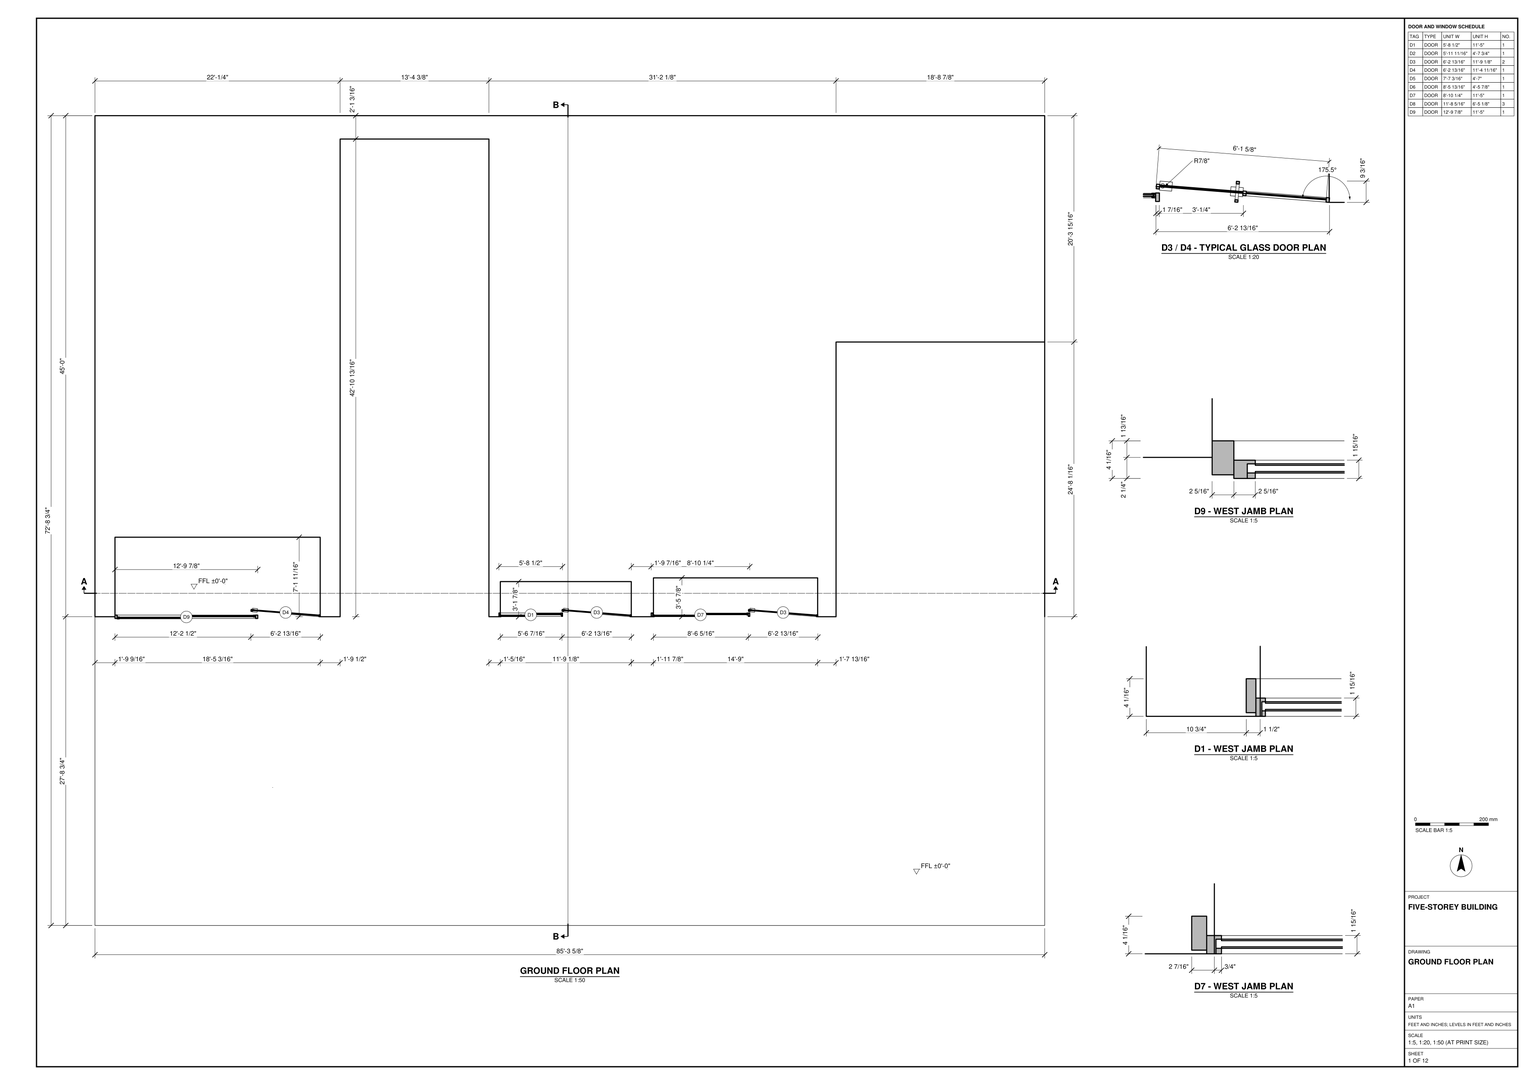
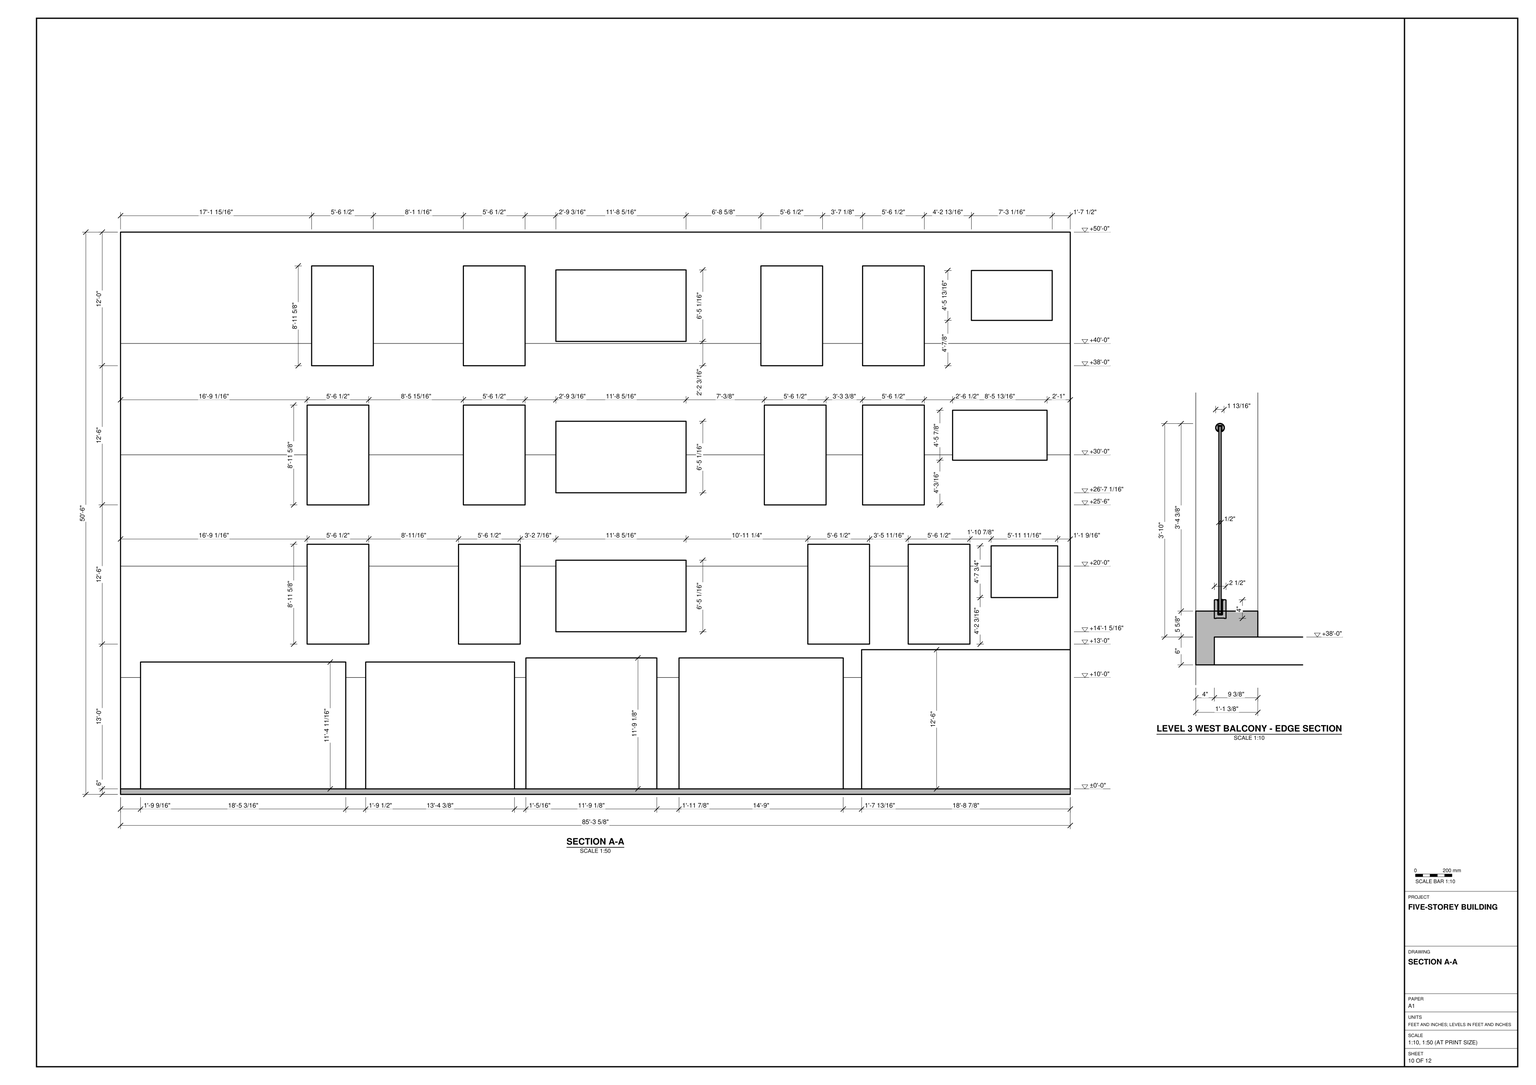
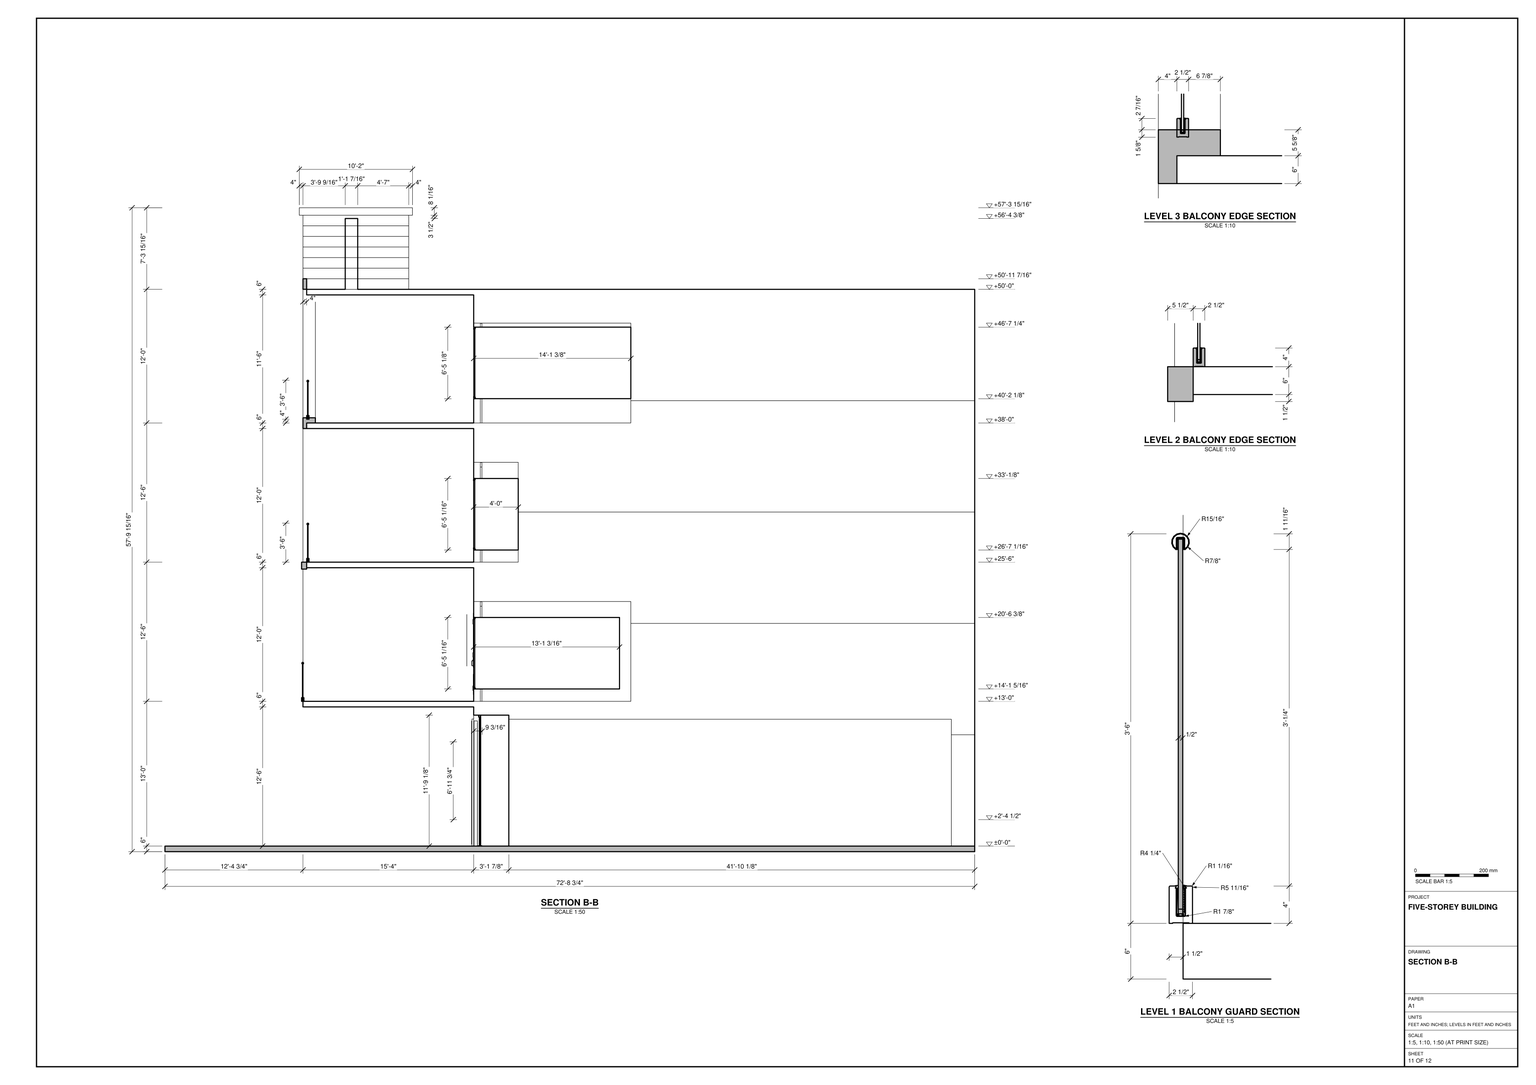
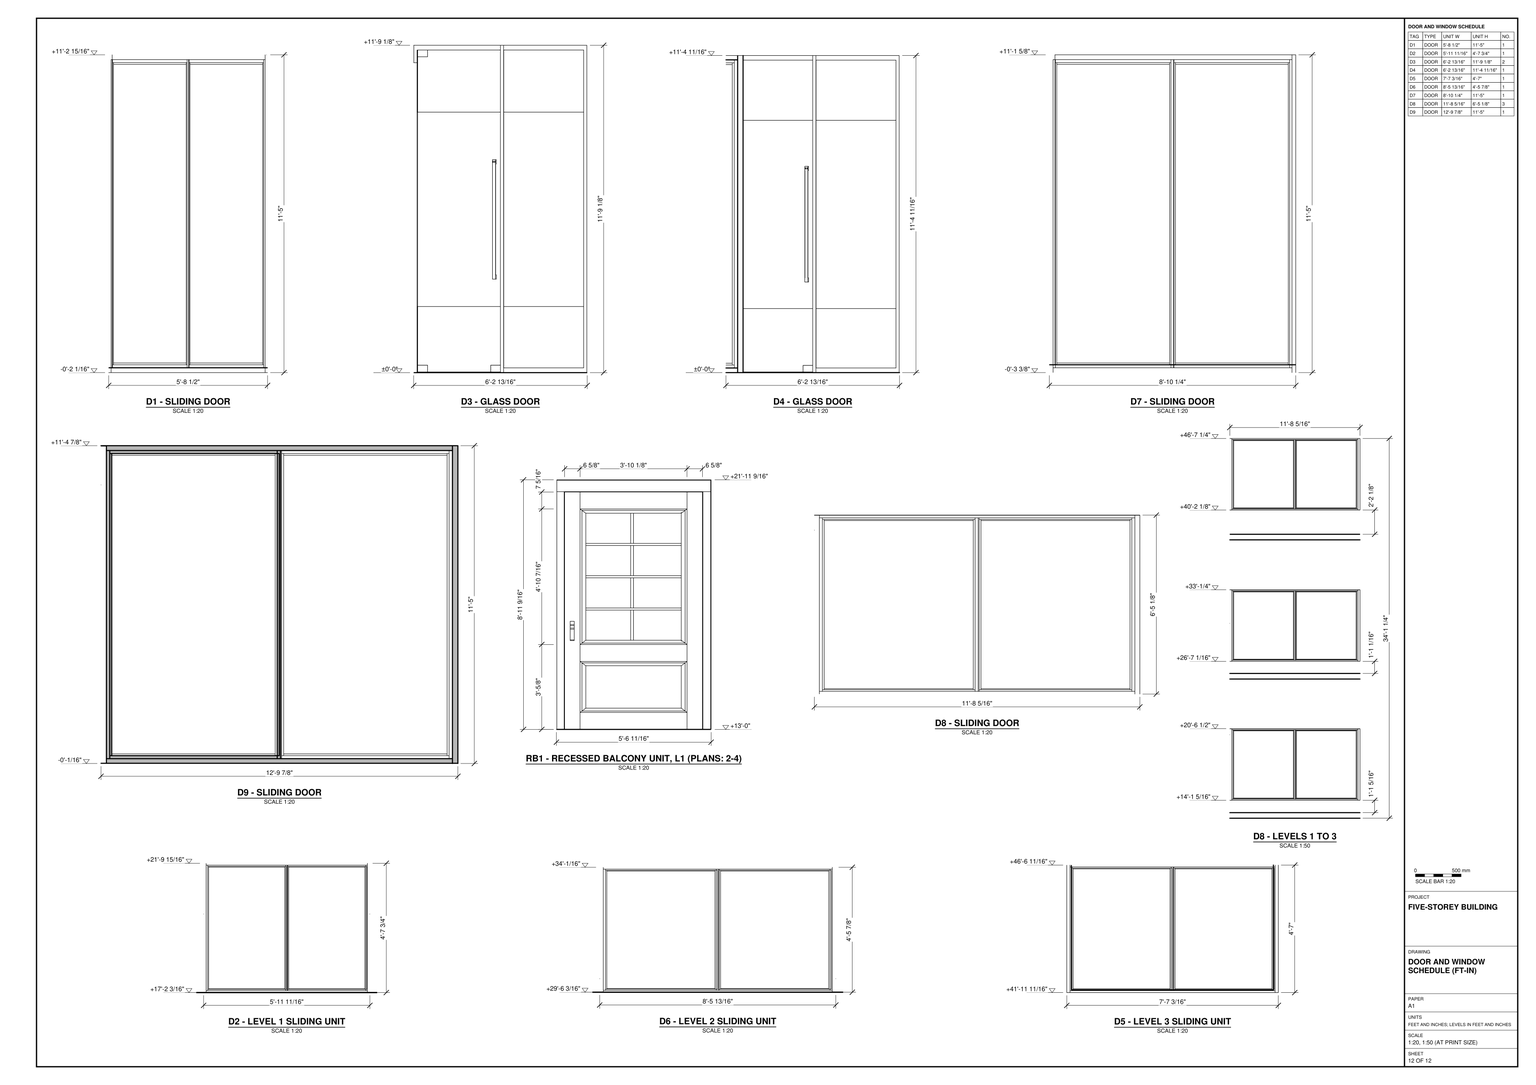
Build the five-storey building in SketchUp from task_files/diagram_01.pdf. Work in feet and inches. The overall model extents are 85'-7 5/8" along X, 72'-8 3/4" along Y and 57'-9 15/16" along Z. Set the ground floor at ±0'-0" and the successive levels at +13'-0", +25'-6", +38'-0" and +50'-0".

Start with the rectangular ground slab. Trace the stepped ground-floor footprint, preserving the deep recess between the entrance bays and the setback at the east end. Model the walls at their drawn thicknesses and fit the glazed door assemblies to the openings using the plan and jamb details. Use section A-A to locate the tall openings and the wider horizontal openings on each upper floor rather than repeating an identical layout. Use section B-B and the enlarged details to shape the projecting balcony slabs, their edges and their glass guards. Include the roof slab and the capped structure rising above it. Follow the plans for any stairs, built-in joinery and main furniture shown.

Keep shell elements and each furniture or joinery piece in separate groups or components, and use components for repeated parts. Decor and loose items may be any suitable library components. Save one SketchUp model as output_files/five_storey_building_with_glazed_entries_and_balconies.skp.

# SketchUp Ruby script. Lengths in inches.
U = 1.inch
M = Sketchup.active_model
def pt(a) = Geom::Point3d.new(a.map { |v| v * U })
def face(e, loops, mat)
  f = e.add_face(loops[0].map { |a| pt(a) })
  loops[1..].each { |l| e.add_face(l.map { |a| pt(a) }).erase! }
  f.material = f.back_material = mat if mat
  f
end
# faces: each face lists its corners as indices into pts; further lists are holes
def faces(e, pts, list, mat = nil) = list.each { |f| face(e, (f[0].is_a?(Array) ? f : [f]).map { |l| l.map { |i| pts[i] } }, mat) }
# xy, xz, yz: faces in a plane at the given z, y or x. An outline is a flat list of corners, or four numbers for a rectangle; further outlines are holes
def ring(l) = l.size == 4 ? [[l[0], l[1]], [l[2], l[1]], [l[2], l[3]], [l[0], l[3]]] : l.each_slice(2).to_a
def flat(e, list, mat, &to3) = list.each { |f| face(e, (f[0].is_a?(Array) ? f : [f]).map { |l| ring(l).map { |u, v| to3.(u, v) } }, mat) }
def xy(e, z, list, mat = nil) = flat(e, list, mat) { |x, y| [x, y, z] }
def xz(e, y, list, mat = nil) = flat(e, list, mat) { |x, z| [x, y, z] }
def yz(e, x, list, mat = nil) = flat(e, list, mat) { |y, z| [x, y, z] }
def lines(e, pts, list) = list.each { |a, b| e.add_line(pt(pts[a]), pt(pts[b])) }
# prism: a flat outline (further loops are holes) pulled along v
def prism(e, loops, v, mat = nil)
  f = face(e, loops, mat); d = Geom::Vector3d.new(v.map { |x| x * U })
  f.pushpull(f.normal.samedirection?(d) ? d.length : -d.length)
end
def box(e, o, s, mat = nil) = prism(e, [[o, [o[0] + s[0], o[1], o[2]], [o[0] + s[0], o[1] + s[1], o[2]], [o[0], o[1] + s[1], o[2]]]], [0, 0, s[2]], mat)
def at(x, y, z, deg = 0) = Geom::Transformation.translation(pt([x, y, z])) * Geom::Transformation.rotation(ORIGIN, Z_AXIS, deg.degrees)
def axes(o, x, y, z) = Geom::Transformation.new([*x, 0, *y, 0, *z, 0, *pt(o).to_a, 1])
def part(name) = M.definitions.add(name)
# library, detail: a bought-in or finely detailed component or shape, given as its bounding box
def library(name, o, s) = part(name).tap { |d| box(d.entities, o, s) }
def detail(e, o, s) = box(e.add_group.entities, o, s)
def put(e, d, t, mat = nil) = e.add_instance(d, t).tap { |i| i.material = mat if mat }
def group(e, t, mat = nil) = e.add_group.tap { |g| g.transformation = t; g.material = mat if mat }.entities
root = M.entities
M.materials.add("Color_B03").color = [113, 96, 78]
M.materials.add("Glass_Tinted_Gray").color = [0, 0, 0]
M.materials["Glass_Tinted_Gray"].alpha = 0.125
M.materials.add("[0135_DarkGray]").color = [81, 81, 81]
M.materials.add("[Color_007]").color = [58, 58, 58]
M.materials.add("[Color_C10]").color = [204, 183, 163]
M.materials.add("[Color_E22]").color = [51, 51, 10]
M.materials.add("[Mirror 02]").color = [229, 229, 229]
M.materials.add("[Terrazzo Light Blue]").color = [196, 214, 227]
M.materials.add("[Wood Floor Parquet]").color = [145, 89, 39]
M.materials.add("[Wood Veneer 01]").color = [120, 70, 37]
c1 = part("Door frame head")
box(c1.entities,[24,0,0],[40,1.75,4],"[Color_C10]")
c2 = part("Door jamb")
box(c2.entities,[0,0,0],[2,1.75,84],"[Color_C10]")
c3 = part("Door panel moulding")
xy(c3.entities,0,[[0,0,47.875,0.25],[0,2,47.875,2.25]],"[Color_C10]")
xy(c3.entities,1.5,[[1.5,0.25,46.375,2]],"[Color_C10]")
xz(c3.entities,0,[[0,0,47.875,0,47.375,0.5,0.5,0.5]],"[Color_C10]")
xz(c3.entities,2.25,[[0,0,0.5,0.5,47.375,0.5,47.875,0]],"[Color_C10]")
p = [[46.375,0.25,1.5],[1.5,0.25,1.5],[0.5,0,0.5],[47.375,0,0.5],[1.5,2,1.5],[46.375,2,1.5],
  [47.375,2.25,0.5],[0.5,2.25,0.5]]
faces(c3.entities,p,[[0,1,2,3],[4,5,6,7]],"[Color_C10]")
c4 = part("Hinge plate")
box(c4.entities,[0,0,0],[0.125,2.5,4],"[Color_E22]")
c5 = part("Door panel moulding \#1")
xy(c5.entities,0,[[0,0,27.75,0.25],[0,2,27.75,2.25]],"[Color_C10]")
xy(c5.entities,1.5,[[1.5,0.25,26.25,2]],"[Color_C10]")
xz(c5.entities,0,[[0,0,27.75,0,27.25,0.5,0.5,0.5]],"[Color_C10]")
xz(c5.entities,2.25,[[0,0,0.5,0.5,27.25,0.5,27.75,0]],"[Color_C10]")
p = [[26.25,0.25,1.5],[1.5,0.25,1.5],[0.5,0,0.5],[27.25,0,0.5],[27.25,2.25,0.5],[0.5,2.25,0.5],
  [1.5,2,1.5],[26.25,2,1.5]]
faces(c5.entities,p,[[0,1,2,3],[4,5,6,7]],"[Color_C10]")
c6 = part("Door pull handle")
xy(c6.entities,0,[[0,0.24,1.05,1.04]],"[Color_E22]")
xy(c6.entities,0.3,[[0,0.64,1.05,1.04]],"[Color_E22]")
xy(c6.entities,6.83,[[0,1.4375,1.05,1.875]],"[Color_E22]")
xz(c6.entities,0,[[0,0.24,1.05,4.01]],"[Color_E22]")
xz(c6.entities,0.39,[[0,0.55,1.05,3.59]],"[Color_E22]")
xz(c6.entities,1.17,[[0,0.07,1.05,0.22]],"[Color_E22]")
xz(c6.entities,1.4375,[[0,5.64,1.05,6.83]],"[Color_E22]")
yz(c6.entities,0,[[0.24,0,0.12,0.03,0.03,0.12,0,0.24,0,4.01,0.02,4.17,0.09,4.31,0.2,4.43,1.28,5.31,1.36,5.4,1.42,5.52,1.4375,5.64,1.4375,6.83,1.875,6.83,1.875,5.29,1.86,5.18,1.81,5.08,1.73,5,0.7,4.22,0.53,4.05,0.43,3.83,0.39,3.59,0.39,0.55,0.42,0.42,0.52,0.33,0.64,0.3,1.04,0.3,1.17,0.22,1.17,0.07,1.04,0]],"[Color_E22]")
yz(c6.entities,1.05,[[0.24,0,1.04,0,1.17,0.07,1.17,0.22,1.04,0.3,0.64,0.3,0.52,0.33,0.42,0.42,0.39,0.55,0.39,3.59,0.43,3.83,0.53,4.05,0.7,4.22,1.73,5,1.81,5.08,1.86,5.18,1.875,5.29,1.875,6.83,1.4375,6.83,1.4375,5.64,1.42,5.52,1.36,5.4,1.28,5.31,0.2,4.43,0.09,4.31,0.02,4.17,0,4.01,0,0.24,0.03,0.12,0.12,0.03]],"[Color_E22]")
p = [[0,0.03,0.12],[0,0.12,0.03],[1.05,0.12,0.03],[1.05,0.03,0.12],[0,0.24,0],[1.05,0.24,0],
  [1.05,1.17,0.07],[1.05,1.04,0],[0,1.04,0],[0,1.17,0.07],[0,0,0.24],[1.05,0,0.24],
  [1.05,1.04,0.3],[1.05,1.17,0.22],[0,1.17,0.22],[0,1.04,0.3],[0,0.52,0.33],[0,0.42,0.42],
  [1.05,0.42,0.42],[1.05,0.52,0.33],[0,0.64,0.3],[1.05,0.64,0.3],[0,0.39,0.55],[1.05,0.39,0.55],
  [0,0.39,3.59],[0,0.43,3.83],[1.05,0.43,3.83],[1.05,0.39,3.59],[0,0.53,4.05],[1.05,0.53,4.05],
  [0,0.02,4.17],[0,0,4.01],[1.05,0,4.01],[1.05,0.02,4.17],[0,0.7,4.22],[1.05,0.7,4.22],
  [0,0.09,4.31],[1.05,0.09,4.31],[0,1.73,5],[1.05,1.73,5],[0,0.2,4.43],[1.05,0.2,4.43],
  [1.05,1.28,5.31],[0,1.28,5.31],[1.05,1.81,5.08],[0,1.81,5.08],[1.05,1.86,5.18],[0,1.86,5.18],
  [1.05,1.875,5.29],[0,1.875,5.29],[0,1.36,5.4],[1.05,1.36,5.4],[0,1.42,5.52],[1.05,1.42,5.52],
  [0,1.4375,5.64],[1.05,1.4375,5.64]]
faces(c6.entities,p,[[0,1,2,3],[1,4,5,2],[6,7,8,9],[10,0,3,11],[12,13,14,15],[16,17,18,19],[20,16,19,21],[17,22,23,18],
  [24,25,26,27],[25,28,29,26],[30,31,32,33],[28,34,35,29],[36,30,33,37],[34,38,39,35],[40,36,37,41],[40,41,42,43],
  [44,39,38,45],[46,44,45,47],[48,46,47,49],[50,43,42,51],[52,50,51,53],[54,52,53,55]],"[Color_E22]")
c7 = part("Component\#153")
xz(c7.entities,0,[[0,6,27.75,53.875]],"[Color_007]")
c8 = part("Door panel moulding \#2")
xy(c8.entities,0,[[35.875,0,53.875,0.25],[35.875,2,53.875,2.25]],"[Color_C10]")
xy(c8.entities,1.5,[[37.375,0.25,52.375,2]],"[Color_C10]")
xz(c8.entities,0,[[35.875,0,53.875,0,53.375,0.5,36.375,0.5]],"[Color_C10]")
xz(c8.entities,2.25,[[35.875,0,36.375,0.5,53.375,0.5,53.875,0]],"[Color_C10]")
p = [[52.375,0.25,1.5],[37.375,0.25,1.5],[36.375,0,0.5],[53.375,0,0.5],[37.375,2,1.5],[52.375,2,1.5],
  [53.375,2.25,0.5],[36.375,2.25,0.5]]
faces(c8.entities,p,[[0,1,2,3],[4,5,6,7]],"[Color_C10]")
c9 = part("Door stile")
box(c9.entities,[0,0,0],[4,1.75,83.875],"[Color_C10]")
c10 = part("Lower door panel")
box(c10.entities,[0,0,0],[27.75,1.75,30],"[Color_C10]")
c11 = part("Door panel moulding \#3")
xy(c11.entities,0,[[0,0,27.75,0.25],[0,2,27.75,2.25]],"[Color_C10]")
xy(c11.entities,1.5,[[1.5,0.25,26.25,2]],"[Color_C10]")
xz(c11.entities,0,[[0,0,27.75,0,27.25,0.5,0.5,0.5]],"[Color_C10]")
xz(c11.entities,2.25,[[0,0,0.5,0.5,27.25,0.5,27.75,0]],"[Color_C10]")
p = [[26.25,0.25,1.5],[1.5,0.25,1.5],[0.5,0,0.5],[27.25,0,0.5],[27.25,2.25,0.5],[0.5,2.25,0.5],
  [1.5,2,1.5],[26.25,2,1.5]]
faces(c11.entities,p,[[0,1,2,3],[4,5,6,7]],"[Color_C10]")
c12 = part("Door rail")
box(c12.entities,[0,0,0],[27.75,1.75,6],"[Color_C10]")
c13 = part("Horizontal glazing bar")
xy(c13.entities,0,[[0,0,24.75,1.75]],"[Color_C10]")
xy(c13.entities,0.75,[[0,0,24.75,1.75]],"[Color_C10]")
xz(c13.entities,0,[[0,0,24.75,0.75]],"[Color_C10]")
xz(c13.entities,1.75,[[0,0,24.75,0.75]],"[Color_C10]")
c14 = part("Vertical glazing bar")
xz(c14.entities,0,[[0,6,0.75,16.66],[0,17.41,0.75,28.0625],[0,28.8125,0.75,39.47],[0,40.22,0.75,50.875]],"[Color_C10]")
xz(c14.entities,1.75,[[0,6,0.75,16.66],[0,17.41,0.75,28.0625],[0,28.8125,0.75,39.47],[0,40.22,0.75,50.875]],"[Color_C10]")
yz(c14.entities,0,[[0,6,1.75,16.66],[0,17.41,1.75,28.0625],[0,28.8125,1.75,39.47],[0,40.22,1.75,50.875]],"[Color_C10]")
yz(c14.entities,0.75,[[0,6,1.75,16.66],[0,17.41,1.75,28.0625],[0,28.8125,1.75,39.47],[0,40.22,1.75,50.875]],"[Color_C10]")
c15 = part("Glazed door leaf")
p = [[5.625,-5.28,31.125],[5.625,-5.28,42.53],[5.625,-5.28,53.9375],[5.625,-5.28,65.34],[5.625,-5.28,76.75]]
lines(c15.entities,p,[[0,1],[1,2],[2,3],[3,4]])
put(c15.entities,c3,axes([4.125,1.625,77.875],[0,0,-1],[0,1,0],[1,0,0]))
put(c15.entities,c4,at(0,1.125,68.3))
put(c15.entities,c5,at(4.125,1.625,6))
put(c15.entities,c6,at(33.38,0,31.375))
put(c15.entities,c7,at(4.125,2.75,24))
put(c15.entities,c8,axes([31.875,1.625,59.875],[0,0,-1],[0,1,0],[-1,0,0]))
put(c15.entities,c9,at(31.875,1.875,0))
put(c15.entities,c8,axes([4.125,1.625,59.875],[0,0,-1],[0,1,0],[1,0,0]))
put(c15.entities,c10,at(4.125,1.875,0))
put(c15.entities,c11,axes([4.125,1.625,77.875],[1,0,0],[0,1,0],[0,0,-1]))
put(c15.entities,c3,axes([31.875,1.625,77.875],[0,0,-1],[0,1,0],[-1,0,0]))
put(c15.entities,c11,at(4.125,1.625,30))
put(c15.entities,c12,at(4.125,1.875,77.875))
put(c15.entities,c9,at(0.125,1.875,0))
put(c15.entities,c13,at(5.625,1.875,42.16))
put(c15.entities,c14,at(18,1.875,25.5))
put(c15.entities,c4,at(0,1.125,9.62))
put(c15.entities,c5,axes([4.125,1.625,24],[1,0,0],[0,1,0],[0,0,-1]))
put(c15.entities,c4,at(0,1.125,38.96))
put(c15.entities,c13,at(5.625,1.875,53.5625))
put(c15.entities,c13,at(5.625,1.875,64.97))
c16 = part("Glazed door assembly")
put(c16.entities,c1,at(-30,0,84))
put(c16.entities,c2,at(32,0,0))
put(c16.entities,c2,at(-6,0,0))
put(c16.entities,c15,axes([32,-1.875,0],[-1,0,0],[0,1,0],[0,0,1]))
c17 = part("PENTEK_RP Fineline 50S_Sliding_DoorCase_E1")
box(c17.entities,[0,0,0],[1.51,3.66,99.27],"[0135_DarkGray]")
c18 = part("PENTEK_RP Fineline 50S_SlidingDooe_Case_E2")
box(c18.entities,[0,0,0],[96.25,3.66,1.51],"[0135_DarkGray]")
c19 = part("pentek_RP Fineline 50S_SlidingDoor_Case")
put(c19.entities,c17,at(97.76,0,0))
put(c19.entities,c18,at(1.51,0,0))
put(c19.entities,c17,at(0,0,0))
put(c19.entities,c18,at(1.51,0,97.76))
c20 = part("PENTEK_RP Fineline 50S_SlidingDoor_GlazingBead_2")
box(c20.entities,[0,0,0],[0.56,0.59,94.39],"[0135_DarkGray]")
c21 = part("PENTEK_RP Fineline 50S_SlidingDoor_Glass")
box(c21.entities,[0,0,0],[46.58,0.16,94.39],"Glass_Tinted_Gray")
c22 = part("PENTEK_RP Fineline 50S_SlidingDoor_GlazingBead")
box(c22.entities,[0,0,0],[45.47,0.59,0.56],"[0135_DarkGray]")
c23 = part("PENTEK_RP Fineline 50S_SlidingDoor_Leaf_E1")
xy(c23.entities,0,[[0,0,0.93,1.97],[0.93,1.57,1.49,1.97]],"[0135_DarkGray]")
xy(c23.entities,96.25,[[0,0,0.93,0,0.93,1.57,1.49,1.57,1.49,1.97,0,1.97]],"[0135_DarkGray]")
xz(c23.entities,0,[[0,0,0.93,96.25]],"[0135_DarkGray]")
xz(c23.entities,1.57,[[0.93,0,1.49,95.32],[0.93,95.32,1.49,96.25]],"[0135_DarkGray]")
xz(c23.entities,1.97,[[0,0,1.49,96.25]],"[0135_DarkGray]")
yz(c23.entities,0,[[0,0,1.97,96.25]],"[0135_DarkGray]")
yz(c23.entities,0.93,[[0,0,1.57,0.93],[0,0.93,1.57,95.32],[0,95.32,1.57,96.25]],"[0135_DarkGray]")
yz(c23.entities,1.49,[[1.57,0,1.97,95.32],[1.57,95.32,1.97,96.25]],"[0135_DarkGray]")
c24 = part("PENTEK_RP Fineline 50S_SlidingDoor_Leaf_E2")
xy(c24.entities,0,[[0,0,0,1.57,0.56,1.57,0.56,1.97,46.02,1.97,46.02,1.57,46.58,1.57,46.58,0]],"[0135_DarkGray]")
xy(c24.entities,0.93,[[0,0,46.58,1.57]],"[0135_DarkGray]")
xy(c24.entities,1.49,[[0.56,1.57,46.02,1.97]],"[0135_DarkGray]")
xz(c24.entities,0,[[0,0,46.58,0.93]],"[0135_DarkGray]")
xz(c24.entities,1.57,[[0,0,0.56,0.93],[46.02,0,46.58,0.93],[0.56,0.93,46.02,1.49]],"[0135_DarkGray]")
xz(c24.entities,1.97,[[0.56,0,46.02,1.49]],"[0135_DarkGray]")
yz(c24.entities,0,[[0,0,1.57,0.93]],"[0135_DarkGray]")
yz(c24.entities,0.56,[[1.57,0,1.97,0.93],[1.57,0.93,1.97,1.49]],"[0135_DarkGray]")
yz(c24.entities,46.02,[[1.57,0,1.97,0.93],[1.57,0.93,1.97,1.49]],"[0135_DarkGray]")
yz(c24.entities,46.58,[[0,0,1.57,0.93]],"[0135_DarkGray]")
c25 = part("PENTEK_RP Fineline S_SlidingDoor_Leaf1")
put(c25.entities,c20,at(0.93,0,0.93))
put(c25.entities,c20,at(46.96,0,0.93))
put(c25.entities,c21,at(1.49,1.42,0.93))
put(c25.entities,c22,at(1.49,0,0.93))
put(c25.entities,c21,at(1.49,0.59,0.93),"[Terrazzo Light Blue]")
put(c25.entities,c23,at(0,0,0))
put(c25.entities,c23,axes([48.44,0,0],[-1,0,0],[0,1,0],[0,0,1]))
put(c25.entities,c24,axes([0.93,0,96.25],[1,0,0],[0,1,0],[0,0,-1]))
put(c25.entities,c24,at(0.93,0,0))
put(c25.entities,c22,at(1.49,0,94.77))
c26 = part("PENTEK_RP Fineline 50S_SlidingDoor_Leaf2")
put(c26.entities,c21,at(1.49,1.42,0.93))
put(c26.entities,c22,at(1.49,0,94.77))
put(c26.entities,c20,at(46.96,0,0.93))
put(c26.entities,c21,at(1.49,0.59,0.93),"[Mirror 02]")
put(c26.entities,c20,at(0.93,0,0.93))
put(c26.entities,c23,at(0,0,0))
put(c26.entities,c23,axes([48.44,0,0],[-1,0,0],[0,1,0],[0,0,1]))
put(c26.entities,c22,at(1.49,0,0.93))
put(c26.entities,c24,axes([0.93,0,96.25],[1,0,0],[0,1,0],[0,0,-1]))
put(c26.entities,c24,at(0.93,0,0))
c27 = part("PENTEK - Slimmest Steel Sliding Door / Window\#1")
put(c27.entities,c19,at(0,-1.88,-0.09))
put(c27.entities,c25,at(1.51,-2.27,1.42))
put(c27.entities,c26,at(49.32,-0.3,1.42))
c28 = library("Glass Rail",[0,0,0],[2.52,48.73,42.05])
c29 = library("door glass6",[-2.49,0,0],[11.76,74.82,94.49])
xy(root,-6,[[4,0,1027.625,872.75]])
xy(root,0,[[4,0,1027.625,0,1027.625,628.8125,802.74,628.8125,802.74,332.75,782.93,332.75,782.93,374.625,605.93,374.625,605.93,332.75,582.04,332.75,582.04,370.625,440.92,370.625,440.92,332.75,428.64,332.75,428.64,847.5625,268.24,847.5625,268.24,332.75,246.74,332.75,246.74,418.4375,25.58,418.4375,25.58,332.75,4,332.75],[4,332.75,25.58,332.75,25.58,418.4375,246.74,418.4375,246.74,332.75,268.24,332.75,268.24,847.5625,428.64,847.5625,428.64,332.75,440.92,332.75,440.92,370.625,582.04,370.625,582.04,332.75,605.93,332.75,605.93,374.625,782.93,374.625,782.93,332.75,802.74,332.75,802.74,628.8125,1027.625,628.8125,1027.625,872.75,4,872.75]])
xy(root,136.6875,[[25.58,332.75,246.74,418.4375],[268.24,332.75,428.64,847.5625]])
xy(root,141.125,[[440.92,332.75,582.04,370.625],[605.93,332.75,782.93,374.625]])
xy(root,150,[[4,148.75,4,332.75,802.74,332.75,802.74,628.8125,1027.625,628.8125,1027.625,148.75]])
xy(root,156,[[535.1,147.25,544.57,148.75],[195.45,148.75,535.1,148.75,535.1,152.75,544.57,152.75,544.57,159.75,711.0625,159.75,711.0625,148.75,1017.75,148.75,1017.75,160.25,1027.625,160.25,1027.625,332.75,919.45,332.75,919.45,502.125,852.95,502.125,852.95,332.75,811.28,332.75,811.28,502.125,744.78,502.125,744.78,332.75,434.78,332.75,434.78,502.125,368.28,502.125,368.28,332.75,271.59,332.75,271.59,502.125,205.09,502.125,205.09,332.75,195.45,332.75],[535.1,148.75,544.57,152.75],[544.57,148.75,694.5,152.75],[694.5,148.75,711.0625,148.75,711.0625,159.75,544.57,159.75,544.57,152.75,694.5,152.75]])
xy(root,169.33,[[473.22,332.75,613.53,489.9375]])
xy(root,206.16,[[942.34,332.75,1014.03,502.125]])
xy(root,246.4,[[473.22,332.75,613.53,489.9375]])
xy(root,261.91,[[942.34,332.75,1014.03,502.125]])
xy(root,263.6,[[205.09,332.75,271.59,502.125],[368.28,332.75,434.78,502.125],[744.78,332.75,811.28,502.125],[852.95,332.75,919.45,502.125]])
xy(root,298.5,[[195.45,147.25,535.1,152.75]],"[Wood Floor Parquet]")
xy(root,300,[[195.45,152.75,195.45,332.75,1027.625,332.75,1027.625,160.25,1017.75,160.25,1017.75,168.0625,948.84,168.0625,948.84,152.75,711.0625,152.75,711.0625,159.75,544.57,159.75,544.57,152.75],[948.84,162,1017.75,168.0625]])
xy(root,306,[[195.45,152.75,544.57,152.75,544.57,158.75,711.0625,158.75,711.0625,152.75,948.84,152.75,948.84,168.0625,1017.75,168.0625,1017.75,154.1875,1027.625,154.1875,1027.625,332.75,870.29,332.75,870.29,380.75,803.79,380.75,803.79,332.75,764.41,332.75,764.41,380.75,697.91,380.75,697.91,332.75,440.03,332.75,440.03,380.75,373.53,380.75,373.53,332.75,271.59,332.75,271.59,380.75,205.09,380.75,205.09,332.75,195.45,332.75]])
xy(root,306,[[195.45,147.25,544.57,152.75]],"[Wood Floor Parquet]")
xy(root,319.08,[[473.22,332.75,613.53,380.75]])
xy(root,342,[[948.84,162,1017.75,168.0625]],"[Wood Floor Parquet]")
xy(root,354.16,[[900.79,332.75,1002.6,380.75]])
xy(root,396.15,[[473.22,332.75,613.53,380.75]])
xy(root,408.03,[[900.79,332.75,1002.6,380.75]])
xy(root,413.6,[[205.09,332.75,271.59,380.75],[373.53,332.75,440.03,380.75],[697.91,332.75,764.41,380.75],[803.79,332.75,870.29,380.75]])
xy(root,450,[[195.45,148.75,544.57,152.75],[195.45,152.75,195.45,332.75,1027.625,332.75,1027.625,154.1875,1017.75,154.1875,1017.75,169.75,948.84,169.75,948.84,152.75,711.0625,152.75,711.0625,158.75,544.57,158.75,544.57,152.75],[948.84,164.4375,1017.75,169.75]])
xy(root,456,[[195.45,152.75,544.57,162.125],[711.0625,152.75,948.84,152.75,948.84,169.75,1017.75,169.75,1017.75,154.1875,1027.625,154.1875,1027.625,332.75,870.29,332.75,870.29,380.75,803.79,380.75,803.79,332.75,760.68,332.75,760.68,380.75,694.18,380.75,694.18,332.75,440.03,332.75,440.03,502.125,373.53,502.125,373.53,332.75,276.47,332.75,276.47,502.125,209.97,502.125,209.97,332.75,195.45,332.75,195.45,162.125,544.57,162.125,544.57,158.75,711.0625,158.75]])
xy(root,461.6,[[244.91,148.75,544.57,162.125]])
xy(root,482.21,[[473.22,332.75,613.53,502.125]])
xy(root,491.5625,[[948.84,164.4375,1017.75,169.75]],"[Wood Floor Parquet]")
xy(root,504.85,[[921.08,332.75,1008.15,386.75]])
xy(root,558.66,[[921.08,332.75,1008.15,386.75]])
xy(root,559.27,[[473.22,332.75,613.53,502.125]])
xy(root,563.6,[[209.97,332.75,276.47,502.125],[373.53,332.75,440.03,502.125],[694.18,332.75,760.68,380.75],[803.79,332.75,870.29,380.75]])
xy(root,594,[[[711.0625,139.5625,711.0625,158.75,544.57,158.75,544.57,152.75,244.91,152.75,244.91,162.125,195.45,162.125,195.45,332.75,1027.625,332.75,1027.625,154.1875,1017.75,154.1875,1017.75,139.5625],[784.6875,156.72,946.4375,194.78]],[195.45,152.75,244.91,162.125],[1017.75,152.75,1027.625,154.1875]])
xy(root,600,[[[711.0625,139.5625,1017.75,139.5625,1017.75,332.75,1027.625,332.75,1027.625,872.75,4,872.75,4,262.75,199,262.75,199,207.75,548.5625,207.75,548.5625,194.28,199,194.28,199,152.75,711.0625,152.75],[784.6875,156.72,946.4375,194.78],[559.3,195.26,558.54,195.36,557.83,195.66,557.22,196.125,556.76,196.73,556.46,197.44,556.36,198.2,556.46,198.96,556.76,199.67,557.22,200.28,557.83,200.75,558.54,201.04,559.3,201.14,560.06,201.04,560.77,200.75,561.375,200.28,561.84,199.67,562.14,198.96,562.24,198.2,562.14,197.44,561.84,196.73,561.375,196.125,560.77,195.66,560.06,195.36],[577.98,195.26,577.22,195.36,576.52,195.66,575.91,196.125,575.44,196.73,575.15,197.44,575.05,198.2,575.15,198.96,575.44,199.67,575.91,200.28,576.52,200.75,577.22,201.04,577.98,201.14,578.74,201.04,579.45,200.75,580.0625,200.28,580.53,199.67,580.82,198.96,580.92,198.2,580.82,197.44,580.53,196.73,580.0625,196.125,579.45,195.66,578.74,195.36],[596.67,195.26,595.91,195.36,595.2,195.66,594.59,196.125,594.125,196.73,593.83,197.44,593.73,198.2,593.83,198.96,594.125,199.67,594.59,200.28,595.2,200.75,595.91,201.04,596.67,201.14,597.43,201.04,598.14,200.75,598.75,200.28,599.21,199.67,599.51,198.96,599.61,198.2,599.51,197.44,599.21,196.73,598.75,196.125,598.14,195.66,597.43,195.36]],[195.45,148.75,199,152.75],[199,148.75,244.91,152.75],[1017.75,152.75,1027.625,332.75]])
xy(root,600.05,[[195.45,148.75,694.5,152.75]])
xy(root,611.4375,[[195.45,148.75,199,152.75],[199,148.75,711.0625,152.75]])
xy(root,676.35,[[[543.5,148.75,543.5,194.28,548.5625,194.28,548.5625,207.75,543.5,207.75,543.5,332.75,1017.75,332.75,1017.75,148.75],[665.97,176.84,963.4,296.78],[559.3,195.26,560.06,195.36,560.77,195.66,561.375,196.125,561.84,196.73,562.14,197.44,562.24,198.2,562.14,198.96,561.84,199.67,561.375,200.28,560.77,200.75,560.06,201.04,559.3,201.14,558.54,201.04,557.83,200.75,557.22,200.28,556.76,199.67,556.46,198.96,556.36,198.2,556.46,197.44,556.76,196.73,557.22,196.125,557.83,195.66,558.54,195.36],[577.98,195.26,578.74,195.36,579.45,195.66,580.0625,196.125,580.53,196.73,580.82,197.44,580.92,198.2,580.82,198.96,580.53,199.67,580.0625,200.28,579.45,200.75,578.74,201.04,577.98,201.14,577.22,201.04,576.52,200.75,575.91,200.28,575.44,199.67,575.15,198.96,575.05,198.2,575.15,197.44,575.44,196.73,575.91,196.125,576.52,195.66,577.22,195.36],[596.67,195.26,597.43,195.36,598.14,195.66,598.75,196.125,599.21,196.73,599.51,197.44,599.61,198.2,599.51,198.96,599.21,199.67,598.75,200.28,598.14,200.75,597.43,201.04,596.67,201.14,595.91,201.04,595.2,200.75,594.59,200.28,594.125,199.67,593.83,198.96,593.73,198.2,593.83,197.44,594.125,196.73,594.59,196.125,595.2,195.66,595.91,195.36]],[543.5,194.28,548.5625,207.75]])
xy(root,676.35,[[199,194.28,543.5,207.75]],"[Wood Veneer 01]")
xy(root,679.875,[[0,144.75,199,148.75],[199,144.75,203,266.75],[0,148.75,4,266.75],[4,148.75,199,262.75],[4,262.75,199,266.75]])
xy(root,686,[[[543.5,148.75,1027.625,332.75],[665.97,176.84,963.4,296.78]]])
xy(root,687.9375,[[0,144.75,203,266.75]])
xz(root,0,[[4,-6,1027.625,0]])
xz(root,139.5625,[[711.0625,594,1017.75,600]])
xz(root,144.75,[[0,679.875,203,687.9375]])
xz(root,147.25,[[535.1,156,544.57,156,544.57,306,195.45,306,195.45,298.5,535.1,298.5]],"[Wood Floor Parquet]")
xz(root,148.75,[[195.45,150,1027.625,150,1027.625,686,543.5,686,543.5,676.35,1017.75,676.35,1017.75,156,195.45,156],[694.5,156,711.0625,156,711.0625,611.4375,195.45,611.4375,195.45,600.05,694.5,600.05],[195.45,450,544.57,450,544.57,461.6,244.91,461.6,244.91,600,195.45,600]])
xz(root,148.75,[[4,150,195.45,150,195.45,611.4375,199,611.4375,199,679.875,4,679.875]],"[0135_DarkGray]")
xz(root,152.75,[[535.1,156,535.1,298.5,195.45,298.5,195.45,300,544.57,300,544.57,156],[195.45,300,544.57,306],[711.0625,300,948.84,306],[195.45,450,544.57,456],[711.0625,450,948.84,456],
  [195.45,594,244.91,600],[244.91,594,544.57,600],[694.5,594,711.0625,600],[1017.75,594,1027.625,600],[195.45,600,199,600.05],
  [694.5,600,694.5,600.05,199,600.05,199,611.4375,711.0625,611.4375,711.0625,600],[195.45,600.05,199,611.4375]])
xz(root,152.75,[[544.57,156,694.5,173.76],[544.57,173.76,694.5,191.52],[544.57,191.52,694.5,209.28],[544.57,209.28,694.5,227.04],[544.57,227.04,694.5,244.8],
  [544.57,244.8,694.5,262.56],[544.57,262.56,694.5,280.32],[544.57,280.32,694.5,298.08],[544.57,298.08,694.5,315.84],[544.57,315.84,694.5,333.6],
  [544.57,333.6,694.5,351.36],[544.57,351.36,694.5,369.12],[544.57,369.12,694.5,386.88],[544.57,386.88,694.5,404.64],[544.57,404.64,694.5,422.4],
  [544.57,422.4,694.5,440.16],[544.57,440.16,694.5,457.92],[544.57,457.92,694.5,475.68],[544.57,475.68,694.5,493.44],[544.57,493.44,694.5,511.2],
  [544.57,511.2,694.5,528.96],[544.57,528.96,694.5,546.72],[544.57,546.72,694.5,564.48],[544.57,564.48,694.5,582.24],[544.57,582.24,694.5,600]],"[0135_DarkGray]")
xz(root,154.1875,[[1017.75,306,1027.625,450],[1017.75,456,1027.625,594]])
xz(root,156.72,[[784.6875,594,946.4375,600]])
xz(root,158.75,[[544.57,306,711.0625,450],[544.57,456,711.0625,594]])
xz(root,159.75,[[544.57,156,711.0625,300]])
xz(root,160.25,[[1017.75,156,1027.625,300]])
xz(root,162,[[948.84,300,1017.75,342]],"[Wood Floor Parquet]")
xz(root,162.125,[[195.45,456,195.45,594,244.91,594,244.91,461.6,544.57,461.6,544.57,456]])
xz(root,164.4375,[[948.84,450,1017.75,491.5625]],"[Wood Floor Parquet]")
xz(root,168.0625,[[948.84,300,1017.75,306]])
xz(root,168.0625,[[948.84,306,1017.75,342]],"[Wood Floor Parquet]")
xz(root,169.75,[[948.84,450,1017.75,456]])
xz(root,169.75,[[948.84,456,1017.75,491.5625]],"[Wood Floor Parquet]")
xz(root,176.84,[[665.97,676.35,963.4,686]])
xz(root,194.28,[[199,610.01,548.5625,610.91],[199,620.91,548.5625,621.8125],[199,631.82,548.5625,632.72],[199,642.73,548.5625,643.63],[199,653.63,548.5625,654.53],
  [199,664.54,548.5625,665.44]],"[0135_DarkGray]")
xz(root,194.28,[[199,600,548.5625,610.01],[199,610.91,548.5625,620.91],[199,621.8125,548.5625,631.82],[199,632.72,548.5625,642.73],[199,643.63,548.5625,653.63],
  [199,654.53,548.5625,664.54],[199,665.44,548.5625,676.35]],"[Wood Veneer 01]")
xz(root,194.78,[[784.6875,594,946.4375,600]])
xz(root,207.75,[[199,600,548.5625,676.35]])
xz(root,262.75,[[4,600,199,679.875]])
xz(root,266.75,[[0,679.875,203,687.9375]])
xz(root,296.78,[[665.97,676.35,963.4,686]])
xz(root,332.75,[[4,0,25.58,0,25.58,136.6875,246.74,136.6875,246.74,0,268.24,0,268.24,136.6875,428.64,136.6875,428.64,0,440.92,0,440.92,141.125,582.04,141.125,582.04,0,605.93,0,605.93,141.125,782.93,141.125,782.93,0,802.74,0,802.74,150,4,150],[[195.45,156,205.09,156,205.09,263.6,271.59,263.6,271.59,156,368.28,156,368.28,263.6,434.78,263.6,434.78,156,744.78,156,744.78,263.6,811.28,263.6,811.28,156,852.95,156,852.95,263.6,919.45,263.6,919.45,156,1027.625,156,1027.625,300,195.45,300],[473.22,169.33,613.53,246.4],[942.34,206.16,1014.03,261.91]],[[195.45,306,205.09,306,205.09,413.6,271.59,413.6,271.59,306,373.53,306,373.53,413.6,440.03,413.6,440.03,306,697.91,306,697.91,413.6,764.41,413.6,764.41,306,803.79,306,803.79,413.6,870.29,413.6,870.29,306,1027.625,306,1027.625,450,195.45,450],[473.22,319.08,613.53,396.15],[900.79,354.16,1002.6,408.03]],[[195.45,456,209.97,456,209.97,563.6,276.47,563.6,276.47,456,373.53,456,373.53,563.6,440.03,563.6,440.03,456,694.18,456,694.18,563.6,760.68,563.6,760.68,456,803.79,456,803.79,563.6,870.29,563.6,870.29,456,1027.625,456,1027.625,594,195.45,594],[473.22,482.21,613.53,559.27],[921.08,504.85,1008.15,558.66]],[1017.75,600,1017.75,676.35,543.5,676.35,543.5,686,1027.625,686,1027.625,600]])
xz(root,370.625,[[440.92,0,582.04,141.125]],"Color_B03")
xz(root,374.625,[[605.93,0,782.93,141.125]])
xz(root,380.75,[[205.09,306,271.59,413.6],[373.53,306,440.03,413.6],[697.91,306,764.41,413.6],[803.79,306,870.29,413.6],[473.22,319.08,613.53,396.15],
  [900.79,354.16,1002.6,408.03],[694.18,456,760.68,563.6],[803.79,456,870.29,563.6]])
xz(root,386.75,[[921.08,504.85,1008.15,558.66]])
xz(root,418.4375,[[25.58,0,246.74,136.6875]])
xz(root,489.9375,[[473.22,169.33,613.53,246.4]])
xz(root,502.125,[[205.09,156,271.59,263.6],[368.28,156,434.78,263.6],[744.78,156,811.28,263.6],[852.95,156,919.45,263.6],[942.34,206.16,1014.03,261.91],
  [209.97,456,276.47,563.6],[373.53,456,440.03,563.6],[473.22,482.21,613.53,559.27]])
xz(root,628.8125,[[802.74,0,1027.625,150]])
xz(root,847.5625,[[268.24,0,428.64,136.6875]])
xz(root,872.75,[[4,-6,1027.625,0],[4,0,1027.625,120],[4,120,1027.625,240],[4,240,1027.625,360],[4,360,1027.625,480],
  [4,480,1027.625,600]])
yz(root,0,[[144.75,679.875,266.75,687.9375]])
yz(root,4,[[0,-6,872.75,0],[332.75,0,872.75,120],[332.75,120,332.75,150,148.75,150,148.75,240,872.75,240,872.75,120],[148.75,240,872.75,360],[148.75,360,872.75,480],
  [148.75,480,872.75,600],[148.75,600,262.75,679.875]])
yz(root,25.58,[[332.75,0,418.4375,136.6875]])
yz(root,195.45,[[148.75,156,332.75,156,332.75,300,152.75,300,152.75,298.5,148.75,298.5],[147.25,298.5,148.75,300],[148.75,298.5,152.75,300],[147.25,300,148.75,306],[148.75,300,152.75,306],
  [148.75,306,332.75,450],[148.75,450,152.75,456],[148.75,456,162.125,594],[162.125,456,332.75,594],[148.75,594,152.75,600],
  [148.75,600,152.75,600.05],[148.75,600.05,152.75,611.4375]])
yz(root,199,[[207.75,600,262.75,611.41],[207.75,611.41,262.75,622.82],[207.75,622.82,262.75,634.23],[207.75,634.23,262.75,645.64],[207.75,645.64,262.75,657.05],
  [207.75,657.05,262.75,668.46]])
yz(root,199,[[152.75,600,194.28,611.41],[152.75,611.41,194.28,611.41,194.28,622.82,148.75,622.82,148.75,611.4375,152.75,611.4375],[148.75,622.82,194.28,634.23],[148.75,634.23,194.28,645.64],[148.75,645.64,194.28,657.05],
  [148.75,657.05,194.28,668.46],[148.75,668.46,194.28,668.46,194.28,676.35,207.75,676.35,207.75,668.46,262.75,668.46,262.75,679.875,148.75,679.875]],"[0135_DarkGray]")
yz(root,203,[[144.75,679.875,266.75,687.9375]])
yz(root,205.09,[[332.75,156,502.125,263.6],[332.75,306,380.75,413.6]])
yz(root,209.97,[[332.75,456,502.125,563.6]])
yz(root,244.91,[[148.75,461.6,162.125,461.6,162.125,594,152.75,594,152.75,600,148.75,600]])
yz(root,246.74,[[332.75,0,418.4375,136.6875]])
yz(root,268.24,[[332.75,0,847.5625,136.6875]])
yz(root,271.59,[[332.75,156,502.125,263.6],[332.75,306,380.75,413.6]])
yz(root,276.47,[[332.75,456,502.125,563.6]])
yz(root,368.28,[[332.75,156,502.125,263.6]])
yz(root,373.53,[[332.75,306,380.75,413.6],[332.75,456,502.125,563.6]])
yz(root,428.64,[[332.75,0,847.5625,136.6875]])
yz(root,434.78,[[332.75,156,502.125,263.6]])
yz(root,440.03,[[332.75,306,380.75,413.6],[332.75,456,502.125,563.6]])
yz(root,440.92,[[332.75,0,370.625,141.125]])
yz(root,473.22,[[332.75,169.33,489.9375,246.4],[332.75,319.08,380.75,396.15],[332.75,482.21,502.125,559.27]])
yz(root,535.1,[[147.25,156,152.75,298.5]],"[Wood Floor Parquet]")
yz(root,543.5,[[148.75,676.35,332.75,686]])
yz(root,544.57,[[152.75,156,159.75,300],[152.75,306,158.75,450],[148.75,450,152.75,461.6],[152.75,456,158.75,461.6],[158.75,456,162.125,461.6],
  [152.75,461.6,158.75,594]])
yz(root,544.57,[[147.25,156,152.75,306]],"[Wood Floor Parquet]")
yz(root,548.5625,[[194.28,600,207.75,676.35]])
yz(root,582.04,[[332.75,0,370.625,141.125]])
yz(root,605.93,[[332.75,0,374.625,141.125]])
yz(root,613.53,[[332.75,169.33,489.9375,246.4],[332.75,319.08,380.75,396.15],[332.75,482.21,502.125,559.27]])
yz(root,665.97,[[176.84,676.35,296.78,686]])
yz(root,694.18,[[332.75,456,380.75,563.6]])
yz(root,694.5,[[148.75,156,152.75,300],[148.75,300,152.75,306],[148.75,306,152.75,600.05]])
yz(root,697.91,[[332.75,306,380.75,413.6]])
yz(root,711.0625,[[148.75,156,159.75,300],[148.75,300,152.75,306],[148.75,306,158.75,450],[148.75,450,152.75,456],[148.75,456,158.75,594],
  [139.5625,594,148.75,600],[148.75,594,152.75,600],[148.75,600,152.75,611.4375]])
yz(root,744.78,[[332.75,156,502.125,263.6]])
yz(root,760.68,[[332.75,456,380.75,563.6]])
yz(root,764.41,[[332.75,306,380.75,413.6]])
yz(root,782.93,[[332.75,0,374.625,141.125]])
yz(root,784.6875,[[156.72,594,194.78,600]])
yz(root,802.74,[[332.75,0,628.8125,150]])
yz(root,803.79,[[332.75,306,380.75,413.6],[332.75,456,380.75,563.6]])
yz(root,811.28,[[332.75,156,502.125,263.6]])
yz(root,852.95,[[332.75,156,502.125,263.6]])
yz(root,870.29,[[332.75,306,380.75,413.6],[332.75,456,380.75,563.6]])
yz(root,900.79,[[332.75,354.16,380.75,408.03]])
yz(root,919.45,[[332.75,156,502.125,263.6]])
yz(root,921.08,[[332.75,504.85,386.75,558.66]])
yz(root,942.34,[[332.75,206.16,502.125,261.91]])
yz(root,946.4375,[[156.72,594,194.78,600]])
yz(root,948.84,[[152.75,300,162,306],[162,300,168.0625,306],[152.75,450,164.4375,456],[164.4375,450,169.75,456]])
yz(root,948.84,[[162,306,168.0625,342],[164.4375,456,169.75,491.5625]],"[Wood Floor Parquet]")
yz(root,963.4,[[176.84,676.35,296.78,686]])
yz(root,1002.6,[[332.75,354.16,380.75,408.03]])
yz(root,1008.15,[[332.75,504.85,386.75,558.66]])
yz(root,1014.03,[[332.75,206.16,502.125,261.91]])
yz(root,1017.75,[[148.75,156,148.75,594,154.1875,594,154.1875,456,164.4375,456,164.4375,450,154.1875,450,154.1875,306,162,306,162,300,160.25,300,160.25,156],[162,300,168.0625,306],[162,306,168.0625,342],[164.4375,450,169.75,456],[164.4375,456,169.75,491.5625],
  [139.5625,594,148.75,600],[148.75,594,152.75,600],[148.75,600,332.75,676.35]])
yz(root,1027.625,[[0,-6,872.75,0],[332.75,0,628.8125,150],[628.8125,0,872.75,0,872.75,600,332.75,600,332.75,156,628.8125,156],[148.75,150,332.75,150,332.75,156,160.25,156,160.25,300,152.75,300,152.75,306,154.1875,306,154.1875,450,152.75,450,152.75,456,154.1875,456,154.1875,594,152.75,594,152.75,600,332.75,600,332.75,686,148.75,686],[332.75,150,628.8125,156],
  [160.25,156,332.75,300],[152.75,300,332.75,306],[154.1875,306,332.75,450],[152.75,450,332.75,456],[154.1875,456,332.75,594],
  [152.75,594,332.75,600]])
# 37 loose lines left out
p = [[558.54,195.36,600],[559.3,195.26,600],[559.3,195.26,676.35],[558.54,195.36,676.35],[560.06,195.36,600],[560.06,195.36,676.35],
  [577.22,195.36,600],[577.98,195.26,600],[577.98,195.26,676.35],[577.22,195.36,676.35],[578.74,195.36,600],[578.74,195.36,676.35],
  [595.91,195.36,600],[596.67,195.26,600],[596.67,195.26,676.35],[595.91,195.36,676.35],[597.43,195.36,600],[597.43,195.36,676.35],
  [557.83,195.66,600],[557.83,195.66,676.35],[560.77,195.66,600],[560.77,195.66,676.35],[576.52,195.66,600],[576.52,195.66,676.35],
  [579.45,195.66,600],[579.45,195.66,676.35],[595.2,195.66,600],[595.2,195.66,676.35],[598.14,195.66,600],[598.14,195.66,676.35],
  [557.22,196.125,600],[557.22,196.125,676.35],[561.375,196.125,600],[561.375,196.125,676.35],[575.91,196.125,600],[575.91,196.125,676.35],
  [580.0625,196.125,600],[580.0625,196.125,676.35],[594.59,196.125,600],[594.59,196.125,676.35],[598.75,196.125,600],[598.75,196.125,676.35],
  [556.76,196.73,600],[556.76,196.73,676.35],[561.84,196.73,600],[561.84,196.73,676.35],[575.44,196.73,600],[575.44,196.73,676.35],
  [580.53,196.73,600],[580.53,196.73,676.35],[594.125,196.73,600],[594.125,196.73,676.35],[599.21,196.73,600],[599.21,196.73,676.35],
  [556.46,197.44,600],[556.46,197.44,676.35],[562.14,197.44,600],[562.14,197.44,676.35],[575.15,197.44,600],[575.15,197.44,676.35],
  [580.82,197.44,600],[580.82,197.44,676.35],[593.83,197.44,600],[593.83,197.44,676.35],[599.51,197.44,600],[599.51,197.44,676.35],
  [556.36,198.2,600],[556.36,198.2,676.35],[562.24,198.2,600],[562.24,198.2,676.35],[575.05,198.2,600],[575.05,198.2,676.35],
  [580.92,198.2,600],[580.92,198.2,676.35],[593.73,198.2,600],[593.73,198.2,676.35],[599.61,198.2,600],[599.61,198.2,676.35],
  [556.46,198.96,600],[556.46,198.96,676.35],[562.14,198.96,600],[562.14,198.96,676.35],[575.15,198.96,600],[575.15,198.96,676.35],
  [580.82,198.96,600],[580.82,198.96,676.35],[593.83,198.96,600],[593.83,198.96,676.35],[599.51,198.96,600],[599.51,198.96,676.35],
  [556.76,199.67,600],[556.76,199.67,676.35],[561.84,199.67,600],[561.84,199.67,676.35],[575.44,199.67,600],[575.44,199.67,676.35],
  [580.53,199.67,600],[580.53,199.67,676.35],[594.125,199.67,600],[594.125,199.67,676.35],[599.21,199.67,600],[599.21,199.67,676.35],
  [557.22,200.28,600],[557.22,200.28,676.35],[561.375,200.28,600],[561.375,200.28,676.35],[575.91,200.28,600],[575.91,200.28,676.35],
  [580.0625,200.28,600],[580.0625,200.28,676.35],[594.59,200.28,600],[594.59,200.28,676.35],[598.75,200.28,600],[598.75,200.28,676.35],
  [557.83,200.75,600],[557.83,200.75,676.35],[560.77,200.75,600],[560.77,200.75,676.35],[576.52,200.75,600],[576.52,200.75,676.35],
  [579.45,200.75,600],[579.45,200.75,676.35],[595.2,200.75,600],[595.2,200.75,676.35],[598.14,200.75,600],[598.14,200.75,676.35],
  [558.54,201.04,600],[558.54,201.04,676.35],[560.06,201.04,600],[560.06,201.04,676.35],[577.22,201.04,600],[577.22,201.04,676.35],
  [578.74,201.04,600],[578.74,201.04,676.35],[595.91,201.04,600],[595.91,201.04,676.35],[597.43,201.04,600],[597.43,201.04,676.35],
  [559.3,201.14,600],[559.3,201.14,676.35],[577.98,201.14,600],[577.98,201.14,676.35],[596.67,201.14,600],[596.67,201.14,676.35]]
faces(root,p,[[0,1,2,3],[1,4,5,2],[6,7,8,9],[7,10,11,8],[12,13,14,15],[13,16,17,14],[18,0,3,19],[4,20,21,5],
  [22,6,9,23],[10,24,25,11],[26,12,15,27],[16,28,29,17],[30,18,19,31],[20,32,33,21],[34,22,23,35],[24,36,37,25],
  [38,26,27,39],[28,40,41,29],[42,30,31,43],[32,44,45,33],[46,34,35,47],[36,48,49,37],[50,38,39,51],[40,52,53,41],
  [54,42,43,55],[44,56,57,45],[58,46,47,59],[48,60,61,49],[62,50,51,63],[52,64,65,53],[66,54,55,67],[56,68,69,57],
  [70,58,59,71],[60,72,73,61],[74,62,63,75],[64,76,77,65],[78,66,67,79],[68,80,81,69],[82,70,71,83],[72,84,85,73],
  [86,74,75,87],[76,88,89,77],[90,78,79,91],[80,92,93,81],[94,82,83,95],[84,96,97,85],[98,86,87,99],[88,100,101,89],
  [102,90,91,103],[92,104,105,93],[106,94,95,107],[96,108,109,97],[110,98,99,111],[100,112,113,101],[114,102,103,115],[104,116,117,105],
  [118,106,107,119],[108,120,121,109],[122,110,111,123],[112,124,125,113],[126,114,115,127],[116,128,129,117],[130,118,119,131],[120,132,133,121],
  [134,122,123,135],[124,136,137,125],[138,126,127,139],[128,138,139,129],[140,130,131,141],[132,140,141,133],[142,134,135,143],[136,142,143,137]])
put(root,c16,axes([215.07,332.5,156],[1.6625,0,0],[0,1,0],[0,0,1.22]))
put(root,c16,axes([215.07,339.91,306],[1.6625,0,0],[0,1,0],[0,0,1.22]))
put(root,c16,axes([219.94,339.91,456],[1.6625,0,0],[0,1,0],[0,0,1.22]))
put(root,c16,axes([383.32,339.91,456],[1.6625,0,0],[0,1,0],[0,0,1.22]))
put(root,c16,axes([383.32,339.91,306],[1.6625,0,0],[0,1,0],[0,0,1.22]))
put(root,c16,axes([378.07,339.91,156],[1.6625,0,0],[0,1,0],[0,0,1.22]))
put(root,c16,axes([754.57,339.91,156],[1.6625,0,0],[0,1,0],[0,0,1.22]))
put(root,c16,axes([862.74,339.91,156],[1.6625,0,0],[0,1,0],[0,0,1.22]))
put(root,c16,axes([813.57,339.91,306],[1.6625,0,0],[0,1,0],[0,0,1.22]))
put(root,c16,axes([707.89,330.75,306],[1.6625,0,0],[0,1,0],[0,0,1.22]))
put(root,c16,axes([704.16,332.75,456],[1.6625,0,0],[0,1,0],[0,0,1.22]))
put(root,c16,axes([813.76,332.75,456],[1.6625,0,0],[0,1,0],[0,0,1.22]))
put(root,c27,axes([473.22,333.75,482.1875],[1.41341,0,0],[0,0.44,0],[0,0,0.77719]))
put(root,c27,axes([473.22,333.58,319.15],[1.41341,0,0],[0,0.44,0],[0,0,0.77719]))
put(root,c27,axes([473.22,333.58,169.4],[1.41341,0,0],[0,0.44,0],[0,0,0.77719]))
put(root,c27,axes([900.79,333.65,354.21],[1.02559,0,0],[0,0.39728,0],[0,0,0.5427]))
put(root,c27,axes([919.08,333.85,503.72],[0.91872,0,0],[0,0.286,0],[0,0,0.55388]))
put(root,c27,axes([942.34,333.65,206.21],[0.72213,0,0],[0,0.39728,0],[0,0,0.56159]))
put(root,c28,axes([195.45,155.27,306],[0,-1,0],[7.16432,0,0],[0,0,1]))
put(root,c28,axes([244.91,155.27,460.02],[0,-1,0],[6.1494,0,0],[0,0,1]))
put(root,c28,axes([710.97,159.04,456],[0,-1,0],[4.88136,0,0],[0,0,1]))
put(root,c28,axes([710.97,159.04,306],[0,-1,0],[4.88136,0,0],[0,0,1]))
put(root,c28,axes([710.97,159.04,156],[0,-1,0],[6.29541,0,0],[0,0,1]))
put(root,c28,axes([185.98,149.77,156],[0,-1,0],[7.16432,0,0],[0,0,1]))
put(root,c29,axes([172.08,341.93,0],[0,-1,0],[1,0,0],[0,0,1.44661]))
put(root,c29,axes([507.375,341.93,0],[0,-1,0],[1,0,0],[0,0,1.49357]))
put(root,c29,axes([708.27,341.93,0],[0,-1,0],[1,0,0],[0,0,1.49357]))
put(root,c27,axes([25.58,332.75,0.03],[1.55,0,0],[0,1,0],[0,0,1.38]))
put(root,c27,axes([439.41,335.02,-1.96],[0.69,0,0],[0,1,0],[0,0,1.38]))
put(root,c27,axes([603.49,335.02,-3.24],[1.07018,0,0],[0,1,0],[0,0,1.38]))
